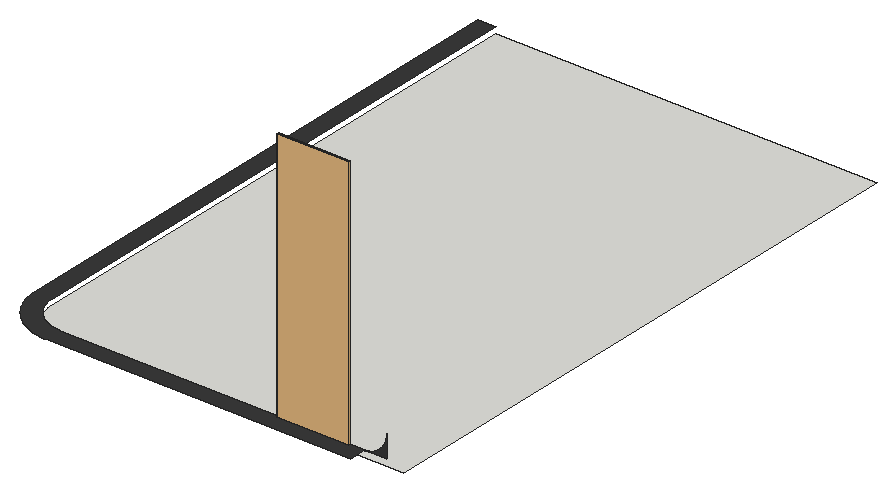
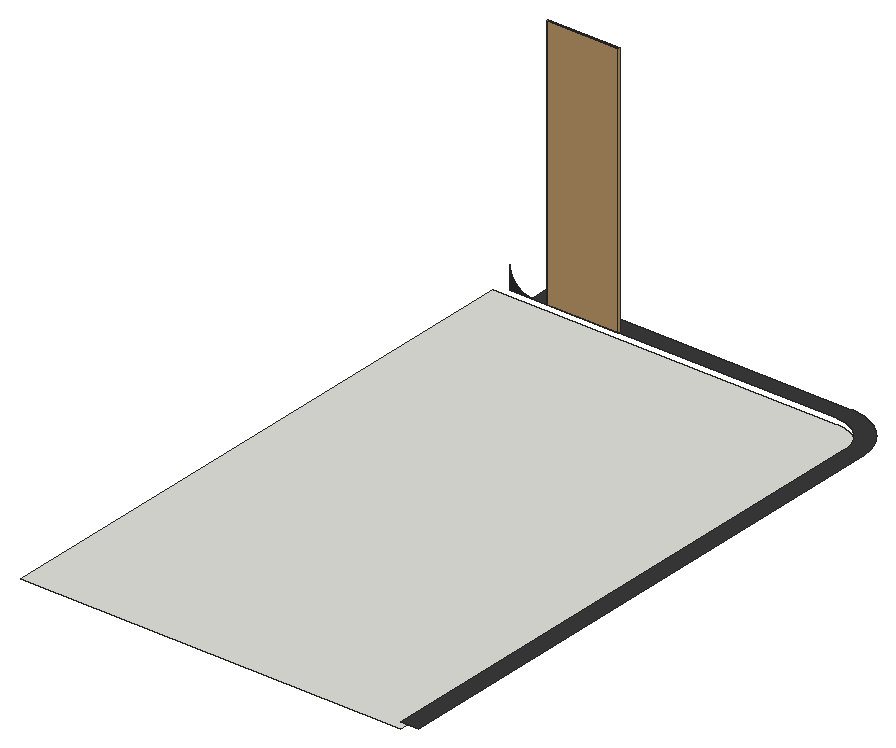
# SketchUp Ruby script. Lengths in inches.
U = 1.inch
M = Sketchup.active_model
def pt(a) = Geom::Point3d.new(a.map { |v| v * U })
def face(e, loops, mat)
  f = e.add_face(loops[0].map { |a| pt(a) })
  loops[1..].each { |l| e.add_face(l.map { |a| pt(a) }).erase! }
  f.material = f.back_material = mat if mat
  f
end
# faces: each face lists its corners as indices into pts; further lists are holes
def faces(e, pts, list, mat = nil) = list.each { |f| face(e, (f[0].is_a?(Array) ? f : [f]).map { |l| l.map { |i| pts[i] } }, mat) }
# xy, xz, yz: faces in a plane at the given z, y or x. An outline is a flat list of corners, or four numbers for a rectangle; further outlines are holes
def ring(l) = l.size == 4 ? [[l[0], l[1]], [l[2], l[1]], [l[2], l[3]], [l[0], l[3]]] : l.each_slice(2).to_a
def flat(e, list, mat, &to3) = list.each { |f| face(e, (f[0].is_a?(Array) ? f : [f]).map { |l| ring(l).map { |u, v| to3.(u, v) } }, mat) }
def xy(e, z, list, mat = nil) = flat(e, list, mat) { |x, y| [x, y, z] }
def xz(e, y, list, mat = nil) = flat(e, list, mat) { |x, z| [x, y, z] }
def yz(e, x, list, mat = nil) = flat(e, list, mat) { |y, z| [x, y, z] }
def lines(e, pts, list) = list.each { |a, b| e.add_line(pt(pts[a]), pt(pts[b])) }
# prism: a flat outline (further loops are holes) pulled along v
def prism(e, loops, v, mat = nil)
  f = face(e, loops, mat); d = Geom::Vector3d.new(v.map { |x| x * U })
  f.pushpull(f.normal.samedirection?(d) ? d.length : -d.length)
end
def box(e, o, s, mat = nil) = prism(e, [[o, [o[0] + s[0], o[1], o[2]], [o[0] + s[0], o[1] + s[1], o[2]], [o[0], o[1] + s[1], o[2]]]], [0, 0, s[2]], mat)
def at(x, y, z, deg = 0) = Geom::Transformation.translation(pt([x, y, z])) * Geom::Transformation.rotation(ORIGIN, Z_AXIS, deg.degrees)
def axes(o, x, y, z) = Geom::Transformation.new([*x, 0, *y, 0, *z, 0, *pt(o).to_a, 1])
def part(name) = M.definitions.add(name)
# library, detail: a bought-in or finely detailed component or shape, given as its bounding box
def library(name, o, s) = part(name).tap { |d| box(d.entities, o, s) }
def detail(e, o, s) = box(e.add_group.entities, o, s)
def put(e, d, t, mat = nil) = e.add_instance(d, t).tap { |i| i.material = mat if mat }
def group(e, t, mat = nil) = e.add_group.tap { |g| g.transformation = t; g.material = mat if mat }.entities
root = M.entities
M.materials.add("1496 AP 8293 CARBON COPY").color = [58, 58, 58]
c1 = library("Group\#16",[0,-1.5,-31],[58,1.5,206])
xy(root,132,[[30.34,119,30.26,119.01,30.1875,119.02,30.11,119.03,29.95,119.05,29.875,119.07,29.8,119.08,29.72,119.1,29.65,119.125,29.57,119.15,29.5,119.17,29.42,119.2,29.21,119.29,29.14,119.33,29.07,119.36,28.93,119.44,28.87,119.48,28.8,119.53,28.74,119.57,28.67,119.62,28.43,119.82,28.38,119.88,28.32,119.93,28.12,120.17,28.07,120.24,28.03,120.3,27.98,120.37,27.94,120.43,27.86,120.57,27.83,120.64,27.79,120.71,27.7,120.92,27.67,121,27.65,121.07,27.625,121.15,27.6,121.22,27.58,121.3,27.57,121.375,27.55,121.45,27.53,121.61,27.52,121.6875,27.51,121.76,27.5,121.84,27.5,122.16,27.51,122.24,27.52,122.3125,27.53,122.39,27.55,122.55,27.57,122.625,27.58,122.7,27.6,122.78,27.625,122.85,27.65,122.93,27.67,123,27.7,123.08,27.79,123.29,27.83,123.36,27.86,123.43,27.94,123.57,27.98,123.63,28.03,123.7,28.07,123.76,28.12,123.83,28.32,124.07,28.38,124.12,28.43,124.18,28.67,124.38,28.74,124.43,28.8,124.47,28.87,124.52,28.93,124.56,29.07,124.64,29.14,124.67,29.21,124.71,29.42,124.8,29.5,124.83,29.57,124.85,29.65,124.875,29.72,124.9,29.8,124.92,29.875,124.93,29.95,124.95,30.11,124.97,30.1875,124.98,30.26,124.99,30.34,125,30.66,125,30.74,124.99,30.8125,124.98,30.89,124.97,31.05,124.95,31.125,124.93,31.2,124.92,31.28,124.9,31.35,124.875,31.43,124.85,31.5,124.83,31.58,124.8,31.79,124.71,31.86,124.67,31.93,124.64,32.07,124.56,32.13,124.52,32.2,124.47,32.26,124.43,32.33,124.38,32.57,124.18,32.62,124.12,32.68,124.07,32.88,123.83,32.93,123.76,32.97,123.7,33.02,123.63,33.06,123.57,33.14,123.43,33.17,123.36,33.21,123.29,33.3,123.08,33.33,123,33.35,122.93,33.375,122.85,33.4,122.78,33.42,122.7,33.43,122.625,33.45,122.55,33.47,122.39,33.48,122.3125,33.49,122.24,33.5,122.16,33.5,121.84,33.49,121.76,33.48,121.6875,33.47,121.61,33.45,121.45,33.43,121.375,33.42,121.3,33.4,121.22,33.375,121.15,33.35,121.07,33.33,121,33.3,120.92,33.21,120.71,33.17,120.64,33.14,120.57,33.06,120.43,33.02,120.37,32.97,120.3,32.93,120.24,32.88,120.17,32.68,119.93,32.62,119.88,32.57,119.82,32.33,119.62,32.26,119.57,32.2,119.53,32.13,119.48,32.07,119.44,31.93,119.36,31.86,119.33,31.79,119.29,31.58,119.2,31.5,119.17,31.43,119.15,31.35,119.125,31.28,119.1,31.2,119.08,31.125,119.07,31.05,119.05,30.89,119.03,30.8125,119.02,30.74,119.01,30.66,119],[100.84,119,100.76,119.01,100.6875,119.02,100.61,119.03,100.45,119.05,100.375,119.07,100.3,119.08,100.22,119.1,100.15,119.125,100.07,119.15,100,119.17,99.92,119.2,99.71,119.29,99.64,119.33,99.57,119.36,99.43,119.44,99.37,119.48,99.3,119.53,99.24,119.57,99.17,119.62,98.93,119.82,98.88,119.88,98.82,119.93,98.62,120.17,98.57,120.24,98.53,120.3,98.48,120.37,98.44,120.43,98.36,120.57,98.33,120.64,98.29,120.71,98.2,120.92,98.17,121,98.15,121.07,98.125,121.15,98.1,121.22,98.08,121.3,98.07,121.375,98.05,121.45,98.03,121.61,98.02,121.6875,98.01,121.76,98,121.84,98,122.16,98.01,122.24,98.02,122.3125,98.03,122.39,98.05,122.55,98.07,122.625,98.08,122.7,98.1,122.78,98.125,122.85,98.15,122.93,98.17,123,98.2,123.08,98.29,123.29,98.33,123.36,98.36,123.43,98.44,123.57,98.48,123.63,98.53,123.7,98.57,123.76,98.62,123.83,98.82,124.07,98.88,124.12,98.93,124.18,99.17,124.38,99.24,124.43,99.3,124.47,99.37,124.52,99.43,124.56,99.57,124.64,99.64,124.67,99.71,124.71,99.92,124.8,100,124.83,100.07,124.85,100.15,124.875,100.22,124.9,100.3,124.92,100.375,124.93,100.45,124.95,100.61,124.97,100.6875,124.98,100.76,124.99,100.84,125,101.16,125,101.24,124.99,101.3125,124.98,101.39,124.97,101.55,124.95,101.625,124.93,101.7,124.92,101.78,124.9,101.85,124.875,101.93,124.85,102,124.83,102.08,124.8,102.29,124.71,102.36,124.67,102.43,124.64,102.57,124.56,102.63,124.52,102.7,124.47,102.76,124.43,102.83,124.38,103.07,124.18,103.12,124.12,103.18,124.07,103.38,123.83,103.43,123.76,103.47,123.7,103.52,123.63,103.56,123.57,103.64,123.43,103.67,123.36,103.71,123.29,103.8,123.08,103.83,123,103.85,122.93,103.875,122.85,103.9,122.78,103.92,122.7,103.93,122.625,103.95,122.55,103.97,122.39,103.98,122.3125,103.99,122.24,104,122.16,104,121.84,103.99,121.76,103.98,121.6875,103.97,121.61,103.95,121.45,103.93,121.375,103.92,121.3,103.9,121.22,103.875,121.15,103.85,121.07,103.83,121,103.8,120.92,103.71,120.71,103.67,120.64,103.64,120.57,103.56,120.43,103.52,120.37,103.47,120.3,103.43,120.24,103.38,120.17,103.18,119.93,103.12,119.88,103.07,119.82,102.83,119.62,102.76,119.57,102.7,119.53,102.63,119.48,102.57,119.44,102.43,119.36,102.36,119.33,102.29,119.29,102.08,119.2,102,119.17,101.93,119.15,101.85,119.125,101.78,119.1,101.7,119.08,101.625,119.07,101.55,119.05,101.39,119.03,101.3125,119.02,101.24,119.01,101.16,119],[199.84,119,199.76,119.01,199.6875,119.02,199.61,119.03,199.45,119.05,199.375,119.07,199.3,119.08,199.22,119.1,199.15,119.125,199.07,119.15,199,119.17,198.92,119.2,198.71,119.29,198.64,119.33,198.57,119.36,198.43,119.44,198.37,119.48,198.3,119.53,198.24,119.57,198.17,119.62,197.93,119.82,197.88,119.88,197.82,119.93,197.62,120.17,197.57,120.24,197.53,120.3,197.48,120.37,197.44,120.43,197.36,120.57,197.33,120.64,197.29,120.71,197.2,120.92,197.17,121,197.15,121.07,197.125,121.15,197.1,121.22,197.08,121.3,197.07,121.375,197.05,121.45,197.03,121.61,197.02,121.6875,197.01,121.76,197,121.84,197,122.16,197.01,122.24,197.02,122.3125,197.03,122.39,197.05,122.55,197.07,122.625,197.08,122.7,197.1,122.78,197.125,122.85,197.15,122.93,197.17,123,197.2,123.08,197.29,123.29,197.33,123.36,197.36,123.43,197.44,123.57,197.48,123.63,197.53,123.7,197.57,123.76,197.62,123.83,197.82,124.07,197.88,124.12,197.93,124.18,198.17,124.38,198.24,124.43,198.3,124.47,198.37,124.52,198.43,124.56,198.57,124.64,198.64,124.67,198.71,124.71,198.92,124.8,199,124.83,199.07,124.85,199.15,124.875,199.22,124.9,199.3,124.92,199.375,124.93,199.45,124.95,199.61,124.97,199.6875,124.98,199.76,124.99,199.84,125,200.16,125,200.24,124.99,200.3125,124.98,200.39,124.97,200.55,124.95,200.625,124.93,200.7,124.92,200.78,124.9,200.85,124.875,200.93,124.85,201,124.83,201.08,124.8,201.29,124.71,201.36,124.67,201.43,124.64,201.57,124.56,201.63,124.52,201.7,124.47,201.76,124.43,201.83,124.38,202.07,124.18,202.12,124.12,202.18,124.07,202.38,123.83,202.43,123.76,202.47,123.7,202.52,123.63,202.56,123.57,202.64,123.43,202.67,123.36,202.71,123.29,202.8,123.08,202.83,123,202.85,122.93,202.875,122.85,202.9,122.78,202.92,122.7,202.93,122.625,202.95,122.55,202.97,122.39,202.98,122.3125,202.99,122.24,203,122.16,203,121.84,202.99,121.76,202.98,121.6875,202.97,121.61,202.95,121.45,202.93,121.375,202.92,121.3,202.9,121.22,202.875,121.15,202.85,121.07,202.83,121,202.8,120.92,202.71,120.71,202.67,120.64,202.64,120.57,202.56,120.43,202.52,120.37,202.47,120.3,202.43,120.24,202.38,120.17,202.18,119.93,202.12,119.88,202.07,119.82,201.83,119.62,201.76,119.57,201.7,119.53,201.63,119.48,201.57,119.44,201.43,119.36,201.36,119.33,201.29,119.29,201.08,119.2,201,119.17,200.93,119.15,200.85,119.125,200.78,119.1,200.7,119.08,200.625,119.07,200.55,119.05,200.39,119.03,200.3125,119.02,200.24,119.01,200.16,119],[298.84,119,298.76,119.01,298.6875,119.02,298.61,119.03,298.45,119.05,298.375,119.07,298.3,119.08,298.22,119.1,298.15,119.125,298.07,119.15,298,119.17,297.92,119.2,297.71,119.29,297.64,119.33,297.57,119.36,297.43,119.44,297.37,119.48,297.3,119.53,297.24,119.57,297.17,119.62,296.93,119.82,296.88,119.88,296.82,119.93,296.62,120.17,296.57,120.24,296.53,120.3,296.48,120.37,296.44,120.43,296.36,120.57,296.33,120.64,296.29,120.71,296.2,120.92,296.17,121,296.15,121.07,296.125,121.15,296.1,121.22,296.08,121.3,296.07,121.375,296.05,121.45,296.03,121.61,296.02,121.6875,296.01,121.76,296,121.84,296,122.16,296.01,122.24,296.02,122.3125,296.03,122.39,296.05,122.55,296.07,122.625,296.08,122.7,296.1,122.78,296.125,122.85,296.15,122.93,296.17,123,296.2,123.08,296.29,123.29,296.33,123.36,296.36,123.43,296.44,123.57,296.48,123.63,296.53,123.7,296.57,123.76,296.62,123.83,296.82,124.07,296.88,124.12,296.93,124.18,297.17,124.38,297.24,124.43,297.3,124.47,297.37,124.52,297.43,124.56,297.57,124.64,297.64,124.67,297.71,124.71,297.92,124.8,298,124.83,298.07,124.85,298.15,124.875,298.22,124.9,298.3,124.92,298.375,124.93,298.45,124.95,298.61,124.97,298.6875,124.98,298.76,124.99,298.84,125,299.16,125,299.24,124.99,299.3125,124.98,299.39,124.97,299.55,124.95,299.625,124.93,299.7,124.92,299.78,124.9,299.85,124.875,299.93,124.85,300,124.83,300.08,124.8,300.29,124.71,300.36,124.67,300.43,124.64,300.57,124.56,300.63,124.52,300.7,124.47,300.76,124.43,300.83,124.38,301.07,124.18,301.12,124.12,301.18,124.07,301.38,123.83,301.43,123.76,301.47,123.7,301.52,123.63,301.56,123.57,301.64,123.43,301.67,123.36,301.71,123.29,301.8,123.08,301.83,123,301.85,122.93,301.875,122.85,301.9,122.78,301.92,122.7,301.93,122.625,301.95,122.55,301.97,122.39,301.98,122.3125,301.99,122.24,302,122.16,302,121.84,301.99,121.76,301.98,121.6875,301.97,121.61,301.95,121.45,301.93,121.375,301.92,121.3,301.9,121.22,301.875,121.15,301.85,121.07,301.83,121,301.8,120.92,301.71,120.71,301.67,120.64,301.64,120.57,301.56,120.43,301.52,120.37,301.47,120.3,301.43,120.24,301.38,120.17,301.18,119.93,301.12,119.88,301.07,119.82,300.83,119.62,300.76,119.57,300.7,119.53,300.63,119.48,300.57,119.44,300.43,119.36,300.36,119.33,300.29,119.29,300.08,119.2,300,119.17,299.93,119.15,299.85,119.125,299.78,119.1,299.7,119.08,299.625,119.07,299.55,119.05,299.39,119.03,299.3125,119.02,299.24,119.01,299.16,119]])
xy(root,138,[[43.61,85,323,85,323,564,14,564,14,114.61,14.01,114.21,14.02,113.82,14.04,113.43,14.0625,113.04,14.09,112.65,14.125,112.25,14.16,111.86,14.26,111.08,14.31,110.7,14.43,109.92,14.5,109.53,14.58,109.15,14.66,108.76,14.74,108.38,14.92,107.62,15.02,107.24,15.125,106.86,15.24,106.48,15.35,106.1,15.59,105.36,15.85,104.62,15.99,104.25,16.14,103.88,16.28,103.52,16.4375,103.16,16.59,102.8,16.76,102.44,16.92,102.08,17.09,101.73,17.45,101.03,17.64,100.69,17.83,100.34,18.02,100,18.22,99.66,18.42,99.33,18.63,98.99,18.84,98.66,19.06,98.33,19.28,98.01,19.5,97.6875,19.73,97.37,19.96,97.05,20.44,96.43,20.6875,96.12,20.93,95.82,21.1875,95.52,21.44,95.22,21.71,94.93,21.97,94.64,22.24,94.35,22.51,94.07,23.07,93.51,23.35,93.24,23.64,92.97,23.93,92.71,24.22,92.44,24.52,92.1875,24.82,91.93,25.12,91.6875,25.43,91.44,26.05,90.96,26.37,90.73,26.6875,90.5,27.01,90.28,27.33,90.06,27.66,89.84,27.99,89.63,28.33,89.42,28.66,89.22,29,89.02,29.34,88.83,29.69,88.64,30.03,88.45,30.73,88.09,31.08,87.92,31.44,87.76,31.8,87.59,32.16,87.4375,32.52,87.28,32.88,87.14,33.25,86.99,33.62,86.85,34.36,86.59,35.1,86.35,35.48,86.24,35.86,86.125,36.24,86.02,36.62,85.92,37.38,85.74,37.76,85.66,38.15,85.58,38.53,85.5,38.92,85.43,39.7,85.31,40.08,85.26,40.86,85.16,41.25,85.125,41.65,85.09,42.04,85.0625,42.43,85.04,42.82,85.02,43.21,85.01]])
xy(root,143,[[43.42,71,291,71,291,85,43.61,85,43.21,85.01,42.82,85.02,42.43,85.04,42.04,85.0625,41.65,85.09,41.25,85.125,40.86,85.16,40.08,85.26,39.7,85.31,38.92,85.43,38.53,85.5,38.15,85.58,37.76,85.66,37.38,85.74,36.62,85.92,36.24,86.02,35.86,86.125,35.48,86.24,35.1,86.35,34.36,86.59,33.62,86.85,33.25,86.99,32.88,87.14,32.52,87.28,32.16,87.4375,31.8,87.59,31.44,87.76,31.08,87.92,30.73,88.09,30.03,88.45,29.69,88.64,29.34,88.83,29,89.02,28.66,89.22,28.33,89.42,27.99,89.63,27.66,89.84,27.33,90.06,27.01,90.28,26.6875,90.5,26.37,90.73,26.05,90.96,25.43,91.44,25.12,91.6875,24.82,91.93,24.52,92.1875,24.22,92.44,23.93,92.71,23.64,92.97,23.35,93.24,23.07,93.51,22.51,94.07,22.24,94.35,21.97,94.64,21.71,94.93,21.44,95.22,21.1875,95.52,20.93,95.82,20.6875,96.12,20.44,96.43,19.96,97.05,19.73,97.37,19.5,97.6875,19.28,98.01,19.06,98.33,18.84,98.66,18.63,98.99,18.42,99.33,18.22,99.66,18.02,100,17.83,100.34,17.64,100.69,17.45,101.03,17.09,101.73,16.92,102.08,16.76,102.44,16.59,102.8,16.4375,103.16,16.28,103.52,16.14,103.88,15.99,104.25,15.85,104.62,15.59,105.36,15.35,106.1,15.24,106.48,15.125,106.86,15.02,107.24,14.92,107.62,14.74,108.38,14.66,108.76,14.58,109.15,14.5,109.53,14.43,109.92,14.31,110.7,14.26,111.08,14.16,111.86,14.125,112.25,14.09,112.65,14.0625,113.04,14.04,113.43,14.02,113.82,14.01,114.21,14,114.61,14,564,0,564,0,114.42,0.02,113.85,0.03,113.27,0.06,112.7,0.09,112.12,0.14,111.55,0.18,110.97,0.3,109.83,0.375,109.26,0.46,108.6875,0.54,108.12,0.74,106.98,0.85,106.42,0.96,105.85,1.08,105.29,1.22,104.73,1.35,104.17,1.5,103.61,1.65,103.06,1.8125,102.5,1.98,101.95,2.15,101.4,2.34,100.86,2.52,100.3125,2.72,99.77,2.92,99.23,3.13,98.7,3.35,98.16,3.57,97.63,3.8,97.1,4.04,96.58,4.54,95.54,4.8,95.02,5.0625,94.51,5.33,94.01,5.61,93.5,5.89,93,6.1875,92.5,6.48,92.01,6.79,91.52,7.1,91.04,7.42,90.55,7.74,90.08,8.4,89.14,8.74,88.67,9.09,88.21,10.17,86.86,10.54,86.42,11.3,85.56,11.69,85.13,12.08,84.71,12.48,84.3,13.3,83.48,13.71,83.08,14.13,82.69,14.56,82.3,15.42,81.54,15.86,81.17,17.21,80.09,17.67,79.74,18.14,79.4,19.08,78.74,19.55,78.42,20.04,78.1,20.52,77.79,21.01,77.48,21.5,77.1875,22,76.89,22.5,76.61,23.01,76.33,23.51,76.0625,24.02,75.8,24.54,75.54,25.58,75.04,26.1,74.8,26.63,74.57,27.16,74.35,27.7,74.13,28.23,73.92,28.77,73.72,29.3125,73.52,29.86,73.34,30.4,73.15,30.95,72.98,31.5,72.8125,32.06,72.65,32.61,72.5,33.17,72.35,33.73,72.22,34.29,72.08,34.85,71.96,35.42,71.85,35.98,71.74,37.12,71.54,37.6875,71.46,38.26,71.375,38.83,71.3,39.97,71.18,40.55,71.14,41.12,71.09,41.7,71.06,42.27,71.03,42.85,71.02]],"1496 AP 8293 CARBON COPY")
xz(root,85,[[291,143,291.24,143,291.47,143.01,291.71,143.01,291.94,143.02,292.18,143.04,292.41,143.06,292.65,143.08,292.88,143.1,293.12,143.125,293.35,143.15,293.58,143.1875,293.82,143.22,294.28,143.3,294.51,143.35,294.74,143.39,294.97,143.44,295.2,143.5,295.43,143.55,295.66,143.61,295.89,143.68,296.11,143.74,296.34,143.81,296.5625,143.88,296.79,143.96,297.01,144.03,297.23,144.11,297.45,144.2,297.67,144.28,298.11,144.46,298.32,144.56,298.54,144.65,298.75,144.75,298.96,144.86,299.17,144.96,299.59,145.18,299.8,145.3,300,145.41,300.4,145.65,300.61,145.78,300.8,145.9,301,146.03,301.2,146.17,301.39,146.3,301.58,146.4375,301.77,146.58,301.96,146.72,302.14,146.86,302.33,147.01,302.51,147.16,302.69,147.3125,302.87,147.47,303.04,147.625,303.22,147.78,303.39,147.94,303.56,148.11,303.73,148.27,303.89,148.44,304.06,148.61,304.22,148.78,304.375,148.96,304.53,149.13,304.6875,149.31,304.84,149.49,304.99,149.67,305.14,149.86,305.28,150.04,305.42,150.23,305.5625,150.42,305.7,150.61,305.83,150.8,305.97,151,306.1,151.2,306.22,151.39,306.35,151.6,306.59,152,306.7,152.2,306.82,152.41,307.04,152.83,307.14,153.04,307.25,153.25,307.35,153.46,307.44,153.68,307.54,153.89,307.72,154.33,307.8,154.55,307.89,154.77,307.97,154.99,308.04,155.21,308.12,155.4375,308.19,155.66,308.26,155.89,308.32,156.11,308.39,156.34,308.45,156.57,308.5,156.8,308.56,157.03,308.61,157.26,308.65,157.49,308.7,157.72,308.78,158.18,308.8125,158.42,308.85,158.65,308.875,158.88,308.9,159.12,308.92,159.35,308.94,159.59,308.96,159.82,308.98,160.06,308.99,160.29,308.99,160.53,309,160.76,309,161,309,143]],"1496 AP 8293 CARBON COPY")
put(root,c1,at(221,85,174))
